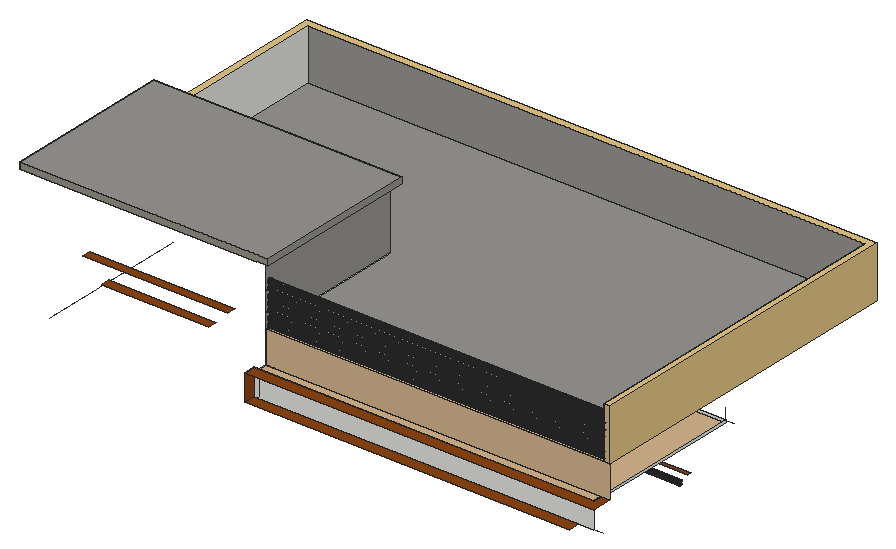
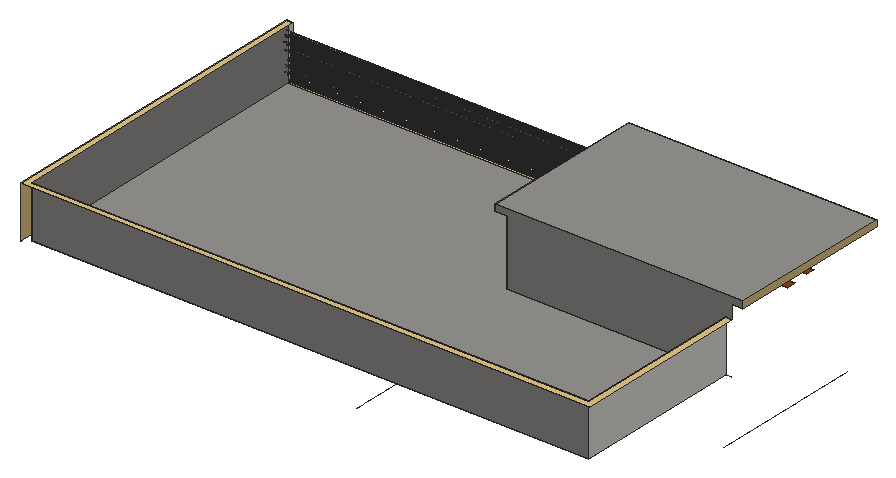
# SketchUp Ruby script. Lengths in inches.
U = 1.inch
M = Sketchup.active_model
def pt(a) = Geom::Point3d.new(a.map { |v| v * U })
def face(e, loops, mat)
  f = e.add_face(loops[0].map { |a| pt(a) })
  loops[1..].each { |l| e.add_face(l.map { |a| pt(a) }).erase! }
  f.material = f.back_material = mat if mat
  f
end
# faces: each face lists its corners as indices into pts; further lists are holes
def faces(e, pts, list, mat = nil) = list.each { |f| face(e, (f[0].is_a?(Array) ? f : [f]).map { |l| l.map { |i| pts[i] } }, mat) }
# xy, xz, yz: faces in a plane at the given z, y or x. An outline is a flat list of corners, or four numbers for a rectangle; further outlines are holes
def ring(l) = l.size == 4 ? [[l[0], l[1]], [l[2], l[1]], [l[2], l[3]], [l[0], l[3]]] : l.each_slice(2).to_a
def flat(e, list, mat, &to3) = list.each { |f| face(e, (f[0].is_a?(Array) ? f : [f]).map { |l| ring(l).map { |u, v| to3.(u, v) } }, mat) }
def xy(e, z, list, mat = nil) = flat(e, list, mat) { |x, y| [x, y, z] }
def xz(e, y, list, mat = nil) = flat(e, list, mat) { |x, z| [x, y, z] }
def yz(e, x, list, mat = nil) = flat(e, list, mat) { |y, z| [x, y, z] }
def lines(e, pts, list) = list.each { |a, b| e.add_line(pt(pts[a]), pt(pts[b])) }
# prism: a flat outline (further loops are holes) pulled along v
def prism(e, loops, v, mat = nil)
  f = face(e, loops, mat); d = Geom::Vector3d.new(v.map { |x| x * U })
  f.pushpull(f.normal.samedirection?(d) ? d.length : -d.length)
end
def box(e, o, s, mat = nil) = prism(e, [[o, [o[0] + s[0], o[1], o[2]], [o[0] + s[0], o[1] + s[1], o[2]], [o[0], o[1] + s[1], o[2]]]], [0, 0, s[2]], mat)
def at(x, y, z, deg = 0) = Geom::Transformation.translation(pt([x, y, z])) * Geom::Transformation.rotation(ORIGIN, Z_AXIS, deg.degrees)
def axes(o, x, y, z) = Geom::Transformation.new([*x, 0, *y, 0, *z, 0, *pt(o).to_a, 1])
def part(name) = M.definitions.add(name)
# library, detail: a bought-in or finely detailed component or shape, given as its bounding box
def library(name, o, s) = part(name).tap { |d| box(d.entities, o, s) }
def detail(e, o, s) = box(e.add_group.entities, o, s)
def put(e, d, t, mat = nil) = e.add_instance(d, t).tap { |i| i.material = mat if mat }
def group(e, t, mat = nil) = e.add_group.tap { |g| g.transformation = t; g.material = mat if mat }.entities
root = M.entities
M.materials.add("[0035_Tan]").color = [210, 180, 140]
M.materials.add("[0043_SaddleBrown]").color = [139, 69, 19]
M.materials.add("[Color M09]").color = [0, 0, 0]
M.materials.add("[Concrete Aggregate Smoke]").color = [154, 150, 148]
M.materials.add("[Formica Graystone]").color = [149, 146, 135]
M.materials.add("[Granite Light Gray]").color = [149, 148, 144]
M.materials.add("[Stone Brushed Khaki]").color = [226, 197, 133]
M.materials.add("[Terrazzo Tile Light]").color = [219, 217, 210]
M.materials.add("[Wood Lumber ButtJoined]").color = [164, 152, 112]
M.materials.add("[Wood Veneer 01]").color = [120, 70, 37]
xy(root,204,[[511.18,244.17,515.23,247.17]])
xy(root,204,[[473.23,244.17,511.18,247.17],[515.23,244.17,557.23,247.17]],"[Wood Veneer 01]")
xy(root,207.54,[[291.78,244.17,385.09,254.42]],"[Concrete Aggregate Smoke]")
xy(root,212.97,[[464.26,244.17,566.2,247.17]],"[Wood Veneer 01]")
xy(root,216.54,[[282.78,244.17,394.09,247.17]],"[Color M09]")
xy(root,248.36,[[244.11,62.42,587.04,74.42]],"[0043_SaddleBrown]")
xy(root,273.75,[[249.49,74.42,249.49,83.42,258.19,83.42,258.19,247.17,603,247.17,603,74.42]],"[0035_Tan]")
xy(root,276,[[249.49,83.42,257.61,247.17],[257.61,83.42,258.19,247.17]])
xy(root,276,[[249.49,74.42,603,83.42]],"[0035_Tan]")
xy(root,276,[[244.11,62.42,612,62.42,612,83.42,603,83.42,603,74.42,244.11,74.42]],"[0043_SaddleBrown]")
xy(root,297.68,[[83.36,74.42,196.9,83.42]],"[0043_SaddleBrown]")
xy(root,310.0625,[[612,83.42,612.4375,434.42]])
xy(root,310.0625,[[249.49,83.42,605.47,89.95]],"[0035_Tan]")
xy(root,310.0625,[[249.49,89.95,605.47,89.95,605.47,427.89,18.53,427.89,18.53,247.17,249.49,247.17]],"[Granite Light Gray]")
xy(root,317.69,[[63.35,74.42,216.91,83.42]],"[0043_SaddleBrown]")
xy(root,364.4375,[[605.47,83.42,612.4375,83.42,612.4375,434.42,12,434.42,12,247.17,18.53,247.17,18.53,427.89,605.47,427.89]],"[Stone Brushed Khaki]")
xy(root,378.52,[[12,71.42,249.49,83.42]],"[Formica Graystone]")
xy(root,378.73,[[0,71.42,12,247.17]],"[Stone Brushed Khaki]")
xy(root,379.14,[[249.49,71.42,261.49,247.17]],"[Granite Light Gray]")
xy(root,385.875,[[0,71.42,261.49,247.17]],"[Granite Light Gray]")
xz(root,71.42,[[12,378.52,249.49,378.52,249.49,379.14,261.49,379.14,261.49,385.875,0,385.875,0,378.73,12,378.73]],"[Formica Graystone]")
xz(root,74.42,[[244.11,248.36,249.49,273.75],[249.49,248.36,603,273.75],[244.11,273.75,249.49,276],[249.49,273.75,603,276]])
xz(root,83.42,[[249.49,273.75,257.61,276],[257.61,273.75,258.19,276]])
xz(root,83.42,[[249.49,276,612,310.0625],[605.47,310.0625,612.4375,364.4375]],"[0035_Tan]")
xz(root,247.17,[[258.19,273.75,603,276]])
xz(root,247.17,[[18.53,310.0625,18.53,364.4375,12,364.4375,12,378.73,0,378.73,0,385.875,261.49,385.875,261.49,379.14,249.49,379.14,249.49,310.0625]],"[Granite Light Gray]")
xz(root,427.89,[[18.53,310.0625,605.47,364.4375]],"[Granite Light Gray]")
yz(root,0,[[71.42,378.73,247.17,385.875]],"[Stone Brushed Khaki]")
yz(root,18.53,[[247.17,310.0625,427.89,364.4375]])
yz(root,244.11,[[62.42,248.36,74.42,276]],"[0043_SaddleBrown]")
yz(root,249.49,[[74.42,273.75,83.42,276],[[83.42,276,247.17,310.0625],[86.63,303.76,86.07,303.83,85.54,304.05,85.09,304.4,84.74,304.85,84.52,305.375,84.45,305.94,84.52,306.51,84.74,307.04,85.09,307.49,85.54,307.84,86.07,308.06,86.63,308.13,87.2,308.06,87.73,307.84,88.18,307.49,88.53,307.04,88.75,306.51,88.82,305.94,88.75,305.375,88.53,304.85,88.18,304.4,87.73,304.05,87.2,303.83],[86.63,296.82,86.07,296.89,85.54,297.11,85.09,297.46,84.74,297.91,84.52,298.4375,84.45,299.01,84.52,299.57,84.74,300.1,85.09,300.55,85.54,300.9,86.07,301.12,86.63,301.19,87.2,301.12,87.73,300.9,88.18,300.55,88.53,300.1,88.75,299.57,88.82,299.01,88.75,298.4375,88.53,297.91,88.18,297.46,87.73,297.11,87.2,296.89]],[86.63,296.82,87.2,296.89,87.73,297.11,88.18,297.46,88.53,297.91,88.75,298.4375,88.82,299.01,88.75,299.57,88.53,300.1,88.18,300.55,87.73,300.9,87.2,301.12,86.63,301.19,86.07,301.12,85.54,300.9,85.09,300.55,84.74,300.1,84.52,299.57,84.45,299.01,84.52,298.4375,84.74,297.91,85.09,297.46,85.54,297.11,86.07,296.89],[86.63,303.76,87.2,303.83,87.73,304.05,88.18,304.4,88.53,304.85,88.75,305.375,88.82,305.94,88.75,306.51,88.53,307.04,88.18,307.49,87.73,307.84,87.2,308.06,86.63,308.13,86.07,308.06,85.54,307.84,85.09,307.49,84.74,307.04,84.52,306.51,84.45,305.94,84.52,305.375,84.74,304.85,85.09,304.4,85.54,304.05,86.07,303.83]])
yz(root,249.49,[[[83.42,310.0625,247.17,310.0625,247.17,379.14,71.42,379.14,71.42,378.52,83.42,378.52],[86.63,345.38,86.07,345.45,85.54,345.67,85.09,346.02,84.74,346.47,84.52,347,84.45,347.57,84.52,348.13,84.74,348.66,85.09,349.11,85.54,349.46,86.07,349.68,86.63,349.76,87.2,349.68,87.73,349.46,88.18,349.11,88.53,348.66,88.75,348.13,88.82,347.57,88.75,347,88.53,346.47,88.18,346.02,87.73,345.67,87.2,345.45],[86.63,338.44,86.07,338.52,85.54,338.74,85.09,339.08,84.74,339.54,84.52,340.0625,84.45,340.63,84.52,341.2,84.74,341.72,85.09,342.18,85.54,342.52,86.07,342.74,86.63,342.82,87.2,342.74,87.73,342.52,88.18,342.18,88.53,341.72,88.75,341.2,88.82,340.63,88.75,340.0625,88.53,339.54,88.18,339.08,87.73,338.74,87.2,338.52],[86.63,331.51,86.07,331.58,85.54,331.8,85.09,332.15,84.74,332.6,84.52,333.125,84.45,333.69,84.52,334.26,84.74,334.79,85.09,335.24,85.54,335.59,86.07,335.81,86.63,335.88,87.2,335.81,87.73,335.59,88.18,335.24,88.53,334.79,88.75,334.26,88.82,333.69,88.75,333.125,88.53,332.6,88.18,332.15,87.73,331.8,87.2,331.58],[86.63,324.57,86.07,324.64,85.54,324.86,85.09,325.21,84.74,325.66,84.52,326.1875,84.45,326.76,84.52,327.32,84.74,327.85,85.09,328.3,85.54,328.65,86.07,328.87,86.63,328.94,87.2,328.87,87.73,328.65,88.18,328.3,88.53,327.85,88.75,327.32,88.82,326.76,88.75,326.1875,88.53,325.66,88.18,325.21,87.73,324.86,87.2,324.64],[86.63,317.63,86.07,317.7,85.54,317.92,85.09,318.27,84.74,318.72,84.52,319.25,84.45,319.82,84.52,320.38,84.74,320.91,85.09,321.36,85.54,321.71,86.07,321.93,86.63,322.01,87.2,321.93,87.73,321.71,88.18,321.36,88.53,320.91,88.75,320.38,88.82,319.82,88.75,319.25,88.53,318.72,88.18,318.27,87.73,317.92,87.2,317.7],[86.63,310.69,86.07,310.77,85.54,310.99,85.09,311.33,84.74,311.79,84.52,312.3125,84.45,312.88,84.52,313.45,84.74,313.97,85.09,314.43,85.54,314.77,86.07,314.99,86.63,315.07,87.2,314.99,87.73,314.77,88.18,314.43,88.53,313.97,88.75,313.45,88.82,312.88,88.75,312.3125,88.53,311.79,88.18,311.33,87.73,310.99,87.2,310.77],[86.63,352.32,86.07,352.39,85.54,352.61,85.09,352.96,84.74,353.41,84.52,353.9375,84.45,354.51,84.52,355.07,84.74,355.6,85.09,356.05,85.54,356.4,86.07,356.62,86.63,356.69,87.2,356.62,87.73,356.4,88.18,356.05,88.53,355.6,88.75,355.07,88.82,354.51,88.75,353.9375,88.53,353.41,88.18,352.96,87.73,352.61,87.2,352.39]]],"[Granite Light Gray]")
yz(root,258.19,[[83.42,273.75,247.17,276]])
yz(root,261.49,[[71.42,379.14,247.17,385.875]],"[Granite Light Gray]")
yz(root,386.65,[[249.32,200.85,249.99,200.94,250.6,201.2,251.14,201.6,251.54,202.13,251.8,202.75,251.89,203.42,251.8,204.08,251.54,204.7,251.14,205.23,250.6,205.63,249.99,205.89,249.32,205.98,248.66,205.89,248.04,205.63,247.51,205.23,247.1,204.7,246.85,204.08,246.76,203.42,246.85,202.75,247.1,202.13,247.51,201.6,248.04,201.2,248.66,200.94]])
yz(root,603,[[74.42,273.75,247.17,276]])
yz(root,605.47,[[83.42,310.0625,89.95,364.4375]])
yz(root,605.47,[[89.95,310.0625,427.89,364.4375]],"[Granite Light Gray]")
yz(root,610.02,[[86.63,310.69,87.2,310.77,87.73,310.99,88.18,311.33,88.53,311.79,88.75,312.3125,88.82,312.88,88.75,313.45,88.53,313.97,88.18,314.43,87.73,314.77,87.2,314.99,86.63,315.07,86.07,314.99,85.54,314.77,85.09,314.43,84.74,313.97,84.52,313.45,84.45,312.88,84.52,312.3125,84.74,311.79,85.09,311.33,85.54,310.99,86.07,310.77],[86.63,317.63,87.2,317.7,87.73,317.92,88.18,318.27,88.53,318.72,88.75,319.25,88.82,319.82,88.75,320.38,88.53,320.91,88.18,321.36,87.73,321.71,87.2,321.93,86.63,322.01,86.07,321.93,85.54,321.71,85.09,321.36,84.74,320.91,84.52,320.38,84.45,319.82,84.52,319.25,84.74,318.72,85.09,318.27,85.54,317.92,86.07,317.7],[86.63,324.57,87.2,324.64,87.73,324.86,88.18,325.21,88.53,325.66,88.75,326.1875,88.82,326.76,88.75,327.32,88.53,327.85,88.18,328.3,87.73,328.65,87.2,328.87,86.63,328.94,86.07,328.87,85.54,328.65,85.09,328.3,84.74,327.85,84.52,327.32,84.45,326.76,84.52,326.1875,84.74,325.66,85.09,325.21,85.54,324.86,86.07,324.64],[86.63,331.51,87.2,331.58,87.73,331.8,88.18,332.15,88.53,332.6,88.75,333.125,88.82,333.69,88.75,334.26,88.53,334.79,88.18,335.24,87.73,335.59,87.2,335.81,86.63,335.88,86.07,335.81,85.54,335.59,85.09,335.24,84.74,334.79,84.52,334.26,84.45,333.69,84.52,333.125,84.74,332.6,85.09,332.15,85.54,331.8,86.07,331.58]])
yz(root,612,[[86.63,338.44,87.2,338.52,87.73,338.74,88.18,339.08,88.53,339.54,88.75,340.0625,88.82,340.63,88.75,341.2,88.53,341.72,88.18,342.18,87.73,342.52,87.2,342.74,86.63,342.82,86.07,342.74,85.54,342.52,85.09,342.18,84.74,341.72,84.52,341.2,84.45,340.63,84.52,340.0625,84.74,339.54,85.09,339.08,85.54,338.74,86.07,338.52],[86.63,345.38,87.2,345.45,87.73,345.67,88.18,346.02,88.53,346.47,88.75,347,88.82,347.57,88.75,348.13,88.53,348.66,88.18,349.11,87.73,349.46,87.2,349.68,86.63,349.76,86.07,349.68,85.54,349.46,85.09,349.11,84.74,348.66,84.52,348.13,84.45,347.57,84.52,347,84.74,346.47,85.09,346.02,85.54,345.67,86.07,345.45],[86.63,352.32,87.2,352.39,87.73,352.61,88.18,352.96,88.53,353.41,88.75,353.9375,88.82,354.51,88.75,355.07,88.53,355.6,88.18,356.05,87.73,356.4,87.2,356.62,86.63,356.69,86.07,356.62,85.54,356.4,85.09,356.05,84.74,355.6,84.52,355.07,84.45,354.51,84.52,353.9375,84.74,353.41,85.09,352.96,85.54,352.61,86.07,352.39]])
yz(root,612.4375,[[83.42,310.0625,434.42,364.4375]],"[Stone Brushed Khaki]")
p = [[473.23,245.22,198.83],[473.23,245.45,198.73],[557.23,245.45,198.73],[557.23,245.22,198.83],[473.23,245.69,198.7],[557.23,245.69,198.7],
  [473.23,245.94,198.73],[557.23,245.94,198.73],[473.23,246.16,198.83],[557.23,246.16,198.83],[473.23,245.03,198.98],[557.23,245.03,198.98],
  [473.23,246.36,198.98],[557.23,246.36,198.98],[473.23,244.88,199.17],[557.23,244.88,199.17],[473.23,246.5,199.17],[557.23,246.5,199.17],
  [473.23,244.79,199.4],[557.23,244.79,199.4],[473.23,246.6,199.4],[557.23,246.6,199.4],[473.23,244.75,199.64],[557.23,244.75,199.64],
  [473.23,246.63,199.64],[557.23,246.63,199.64],[473.23,244.79,199.88],[557.23,244.79,199.88],[473.23,246.6,199.88],[557.23,246.6,199.88],
  [473.23,244.88,200.11],[557.23,244.88,200.11],[473.23,246.5,200.11],[557.23,246.5,200.11],[473.23,245.03,200.3],[557.23,245.03,200.3],
  [473.23,246.36,200.3],[557.23,246.36,200.3],[473.23,245.22,200.45],[557.23,245.22,200.45],[473.23,246.16,200.45],[557.23,246.16,200.45],
  [473.23,245.45,200.54],[557.23,245.45,200.54],[473.23,245.69,200.58],[557.23,245.69,200.58],[473.23,245.94,200.54],[557.23,245.94,200.54],
  [291.78,248.04,201.2],[291.78,248.66,200.94],[386.65,248.66,200.94],[386.65,248.04,201.2],[291.78,249.32,200.85],[386.65,249.32,200.85],
  [291.78,249.99,200.94],[386.65,249.99,200.94],[291.78,250.6,201.2],[386.65,250.6,201.2],[291.78,247.51,201.6],[386.65,247.51,201.6],
  [291.78,251.14,201.6],[386.65,251.14,201.6],[473.23,245.22,201.58],[473.23,245.45,201.48],[557.23,245.45,201.48],[557.23,245.22,201.58],
  [473.23,245.69,201.45],[557.23,245.69,201.45],[473.23,245.94,201.48],[557.23,245.94,201.48],[473.23,246.16,201.58],[557.23,246.16,201.58],
  [473.23,245.03,201.73],[557.23,245.03,201.73],[473.23,246.36,201.73],[557.23,246.36,201.73],[291.78,247.1,202.13],[386.65,247.1,202.13],
  [291.78,251.54,202.13],[386.65,251.54,202.13],[473.23,244.88,201.92],[557.23,244.88,201.92],[473.23,246.5,201.92],[557.23,246.5,201.92],
  [473.23,244.79,202.15],[557.23,244.79,202.15],[473.23,246.6,202.15],[557.23,246.6,202.15],[473.23,244.75,202.39],[557.23,244.75,202.39],
  [473.23,246.63,202.39],[557.23,246.63,202.39],[291.78,246.85,202.75],[386.65,246.85,202.75],[291.78,251.8,202.75],[386.65,251.8,202.75],
  [473.23,244.79,202.63],[557.23,244.79,202.63],[473.23,246.6,202.63],[557.23,246.6,202.63],[473.23,244.88,202.86],[557.23,244.88,202.86],
  [473.23,246.5,202.86],[557.23,246.5,202.86],[291.78,246.76,203.42],[386.65,246.76,203.42],[291.78,251.89,203.42],[386.65,251.89,203.42],
  [473.23,245.03,203.05],[557.23,245.03,203.05],[473.23,246.36,203.05],[557.23,246.36,203.05],[473.23,245.22,203.2],[557.23,245.22,203.2],
  [473.23,246.16,203.2],[557.23,246.16,203.2],[473.23,245.45,203.29],[557.23,245.45,203.29],[473.23,245.94,203.29],[557.23,245.94,203.29],
  [473.23,245.69,203.33],[557.23,245.69,203.33],[291.78,246.85,204.08],[386.65,246.85,204.08],[291.78,251.8,204.08],[386.65,251.8,204.08],
  [291.78,247.1,204.7],[386.65,247.1,204.7],[291.78,251.54,204.7],[386.65,251.54,204.7],[291.78,247.51,205.23],[386.65,247.51,205.23],
  [291.78,251.14,205.23],[386.65,251.14,205.23],[291.78,248.04,205.63],[386.65,248.04,205.63],[291.78,250.6,205.63],[386.65,250.6,205.63],
  [291.78,248.66,205.89],[386.65,248.66,205.89],[291.78,249.99,205.89],[386.65,249.99,205.89],[291.78,249.32,205.98],[386.65,249.32,205.98],
  [339.9,244.17,207.54],[338.43,244.17,207.54],[337.18,244.17,207.54],[337.18,241.18,207.41],[339.9,241.18,207.41],[249.49,86.07,310.77],
  [249.49,86.63,310.69],[610.02,86.63,310.69],[610.02,86.07,310.77],[249.49,87.2,310.77],[610.02,87.2,310.77],[249.49,85.54,310.99],
  [610.02,85.54,310.99],[249.49,87.73,310.99],[610.02,87.73,310.99],[249.49,85.09,311.33],[610.02,85.09,311.33],[249.49,88.18,311.33],
  [610.02,88.18,311.33],[249.49,84.74,311.79],[610.02,84.74,311.79],[249.49,88.53,311.79],[610.02,88.53,311.79],[249.49,84.52,312.3125],
  [610.02,84.52,312.3125],[249.49,88.75,312.3125],[610.02,88.75,312.3125],[249.49,84.45,312.88],[610.02,84.45,312.88],[249.49,88.82,312.88],
  [610.02,88.82,312.88],[249.49,84.52,313.45],[610.02,84.52,313.45],[249.49,88.75,313.45],[610.02,88.75,313.45],[249.49,84.74,313.97],
  [610.02,84.74,313.97],[249.49,88.53,313.97],[610.02,88.53,313.97],[249.49,85.09,314.43],[610.02,85.09,314.43],[249.49,88.18,314.43],
  [610.02,88.18,314.43],[249.49,85.54,314.77],[610.02,85.54,314.77],[249.49,87.73,314.77],[610.02,87.73,314.77],[249.49,86.07,314.99],
  [610.02,86.07,314.99],[249.49,87.2,314.99],[610.02,87.2,314.99],[249.49,86.63,315.07],[610.02,86.63,315.07],[249.49,86.07,317.7],
  [249.49,86.63,317.63],[610.02,86.63,317.63],[610.02,86.07,317.7],[249.49,87.2,317.7],[610.02,87.2,317.7],[249.49,85.54,317.92],
  [610.02,85.54,317.92],[249.49,87.73,317.92],[610.02,87.73,317.92],[249.49,85.09,318.27],[610.02,85.09,318.27],[249.49,88.18,318.27],
  [610.02,88.18,318.27],[249.49,84.74,318.72],[610.02,84.74,318.72],[249.49,88.53,318.72],[610.02,88.53,318.72],[249.49,84.52,319.25],
  [610.02,84.52,319.25],[249.49,88.75,319.25],[610.02,88.75,319.25],[249.49,84.45,319.82],[610.02,84.45,319.82],[249.49,88.82,319.82],
  [610.02,88.82,319.82],[249.49,84.52,320.38],[610.02,84.52,320.38],[249.49,88.75,320.38],[610.02,88.75,320.38],[249.49,84.74,320.91],
  [610.02,84.74,320.91],[249.49,88.53,320.91],[610.02,88.53,320.91],[249.49,85.09,321.36],[610.02,85.09,321.36],[249.49,88.18,321.36],
  [610.02,88.18,321.36],[249.49,85.54,321.71],[610.02,85.54,321.71],[249.49,87.73,321.71],[610.02,87.73,321.71],[249.49,86.07,321.93],
  [610.02,86.07,321.93],[249.49,87.2,321.93],[610.02,87.2,321.93],[249.49,86.63,322.01],[610.02,86.63,322.01],[249.49,85.54,324.86],
  [249.49,86.07,324.64],[610.02,86.07,324.64],[610.02,85.54,324.86],[249.49,86.63,324.57],[610.02,86.63,324.57],[249.49,87.2,324.64],
  [610.02,87.2,324.64],[249.49,87.73,324.86],[610.02,87.73,324.86],[249.49,85.09,325.21],[610.02,85.09,325.21],[249.49,88.18,325.21],
  [610.02,88.18,325.21],[249.49,84.74,325.66],[610.02,84.74,325.66],[249.49,88.53,325.66],[610.02,88.53,325.66],[249.49,84.52,326.1875],
  [610.02,84.52,326.1875],[249.49,88.75,326.1875],[610.02,88.75,326.1875],[249.49,84.45,326.76],[610.02,84.45,326.76],[249.49,88.82,326.76],
  [610.02,88.82,326.76],[249.49,84.52,327.32],[610.02,84.52,327.32],[249.49,88.75,327.32],[610.02,88.75,327.32],[249.49,84.74,327.85],
  [610.02,84.74,327.85],[249.49,88.53,327.85],[610.02,88.53,327.85],[249.49,85.09,328.3],[610.02,85.09,328.3],[249.49,88.18,328.3],
  [610.02,88.18,328.3],[249.49,85.54,328.65],[610.02,85.54,328.65],[249.49,87.73,328.65],[610.02,87.73,328.65],[249.49,86.07,328.87],
  [610.02,86.07,328.87],[249.49,87.2,328.87],[610.02,87.2,328.87],[249.49,86.63,328.94],[610.02,86.63,328.94],[249.49,86.07,331.58],
  [249.49,86.63,331.51],[610.02,86.63,331.51],[610.02,86.07,331.58],[249.49,87.2,331.58],[610.02,87.2,331.58],[249.49,85.54,331.8],
  [610.02,85.54,331.8],[249.49,87.73,331.8],[610.02,87.73,331.8],[249.49,85.09,332.15],[610.02,85.09,332.15],[249.49,88.18,332.15],
  [610.02,88.18,332.15],[249.49,84.74,332.6],[610.02,84.74,332.6],[249.49,88.53,332.6],[610.02,88.53,332.6],[249.49,84.52,333.125],
  [610.02,84.52,333.125],[249.49,88.75,333.125],[610.02,88.75,333.125],[249.49,84.45,333.69],[610.02,84.45,333.69],[249.49,88.82,333.69],
  [610.02,88.82,333.69],[249.49,84.52,334.26],[610.02,84.52,334.26],[249.49,88.75,334.26],[610.02,88.75,334.26],[249.49,84.74,334.79],
  [610.02,84.74,334.79],[249.49,88.53,334.79],[610.02,88.53,334.79],[249.49,85.09,335.24],[610.02,85.09,335.24],[249.49,88.18,335.24],
  [610.02,88.18,335.24],[249.49,85.54,335.59],[610.02,85.54,335.59],[249.49,87.73,335.59],[610.02,87.73,335.59],[249.49,86.07,335.81],
  [610.02,86.07,335.81],[249.49,87.2,335.81],[610.02,87.2,335.81],[249.49,86.63,335.88],[610.02,86.63,335.88],[249.49,86.07,338.52],
  [249.49,86.63,338.44],[612,86.63,338.44],[612,86.07,338.52],[249.49,87.2,338.52],[612,87.2,338.52],[249.49,85.54,338.74],
  [612,85.54,338.74],[249.49,87.73,338.74],[612,87.73,338.74],[249.49,85.09,339.08],[612,85.09,339.08],[249.49,88.18,339.08],
  [612,88.18,339.08],[249.49,84.74,339.54],[612,84.74,339.54],[249.49,88.53,339.54],[612,88.53,339.54],[249.49,84.52,340.0625],
  [612,84.52,340.0625],[249.49,88.75,340.0625],[612,88.75,340.0625],[249.49,84.45,340.63],[612,84.45,340.63],[249.49,88.82,340.63],
  [612,88.82,340.63],[249.49,84.52,341.2],[612,84.52,341.2],[249.49,88.75,341.2],[612,88.75,341.2],[249.49,84.74,341.72],
  [612,84.74,341.72],[249.49,88.53,341.72],[612,88.53,341.72],[249.49,85.09,342.18],[612,85.09,342.18],[249.49,88.18,342.18],
  [612,88.18,342.18],[249.49,85.54,342.52],[612,85.54,342.52],[249.49,87.73,342.52],[612,87.73,342.52],[249.49,86.07,342.74],
  [612,86.07,342.74],[249.49,87.2,342.74],[612,87.2,342.74],[249.49,86.63,342.82],[612,86.63,342.82],[249.49,86.07,345.45],
  [249.49,86.63,345.38],[612,86.63,345.38],[612,86.07,345.45],[249.49,87.2,345.45],[612,87.2,345.45],[249.49,85.54,345.67],
  [612,85.54,345.67],[249.49,87.73,345.67],[612,87.73,345.67],[249.49,85.09,346.02],[612,85.09,346.02],[249.49,88.18,346.02],
  [612,88.18,346.02],[249.49,84.74,346.47],[612,84.74,346.47],[249.49,88.53,346.47],[612,88.53,346.47],[249.49,84.52,347],
  [612,84.52,347],[249.49,88.75,347],[612,88.75,347],[249.49,84.45,347.57],[612,84.45,347.57],[249.49,88.82,347.57],
  [612,88.82,347.57],[249.49,84.52,348.13],[612,84.52,348.13],[249.49,88.75,348.13],[612,88.75,348.13],[249.49,84.74,348.66],
  [612,84.74,348.66],[249.49,88.53,348.66],[612,88.53,348.66],[249.49,85.09,349.11],[612,85.09,349.11],[249.49,88.18,349.11],
  [612,88.18,349.11],[249.49,85.54,349.46],[612,85.54,349.46],[249.49,87.73,349.46],[612,87.73,349.46],[249.49,86.07,349.68],
  [612,86.07,349.68],[249.49,87.2,349.68],[612,87.2,349.68],[249.49,86.63,349.76],[612,86.63,349.76],[249.49,86.07,352.39],
  [249.49,86.63,352.32],[612,86.63,352.32],[612,86.07,352.39],[249.49,87.2,352.39],[612,87.2,352.39],[249.49,85.54,352.61],
  [612,85.54,352.61],[249.49,87.73,352.61],[612,87.73,352.61],[249.49,85.09,352.96],[612,85.09,352.96],[249.49,88.18,352.96],
  [612,88.18,352.96],[249.49,84.74,353.41],[612,84.74,353.41],[249.49,88.53,353.41],[612,88.53,353.41],[249.49,84.52,353.9375],
  [612,84.52,353.9375],[249.49,88.75,353.9375],[612,88.75,353.9375],[249.49,84.45,354.51],[612,84.45,354.51],[249.49,88.82,354.51],
  [612,88.82,354.51],[249.49,84.52,355.07],[612,84.52,355.07],[249.49,88.75,355.07],[612,88.75,355.07],[249.49,84.74,355.6],
  [612,84.74,355.6],[249.49,88.53,355.6],[612,88.53,355.6],[249.49,85.09,356.05],[612,85.09,356.05],[249.49,88.18,356.05],
  [612,88.18,356.05],[249.49,85.54,356.4],[612,85.54,356.4],[249.49,87.73,356.4],[612,87.73,356.4],[249.49,86.07,356.62],
  [612,86.07,356.62],[249.49,87.2,356.62],[612,87.2,356.62],[249.49,86.63,356.69],[612,86.63,356.69],[603,74.42,248.36],
  [612,74.42,248.36],[603,247.17,288],[603,247.17,276],[612,247.17,276],[250.05,83.42,288],[250.05,83.42,276],
  [21,247.17,240],[21,83.42,240],[258.19,247.17,276],[258.19,434.42,276],[18.53,247.17,310.0625],[12,247.17,310.0625]]
faces(root,p,[[0,1,2,3],[1,4,5,2],[4,6,7,5],[6,8,9,7],[10,0,3,11],[8,12,13,9],[14,10,11,15],[12,16,17,13],
  [18,14,15,19],[16,20,21,17],[22,18,19,23],[20,24,25,21],[26,22,23,27],[24,28,29,25],[30,26,27,31],[28,32,33,29],
  [34,30,31,35],[32,36,37,33],[38,34,35,39],[36,40,41,37],[42,38,39,43],[44,42,43,45],[46,44,45,47],[40,46,47,41],
  [62,63,64,65],[63,66,67,64],[66,68,69,67],[68,70,71,69],[72,62,65,73],[70,74,75,71],[80,72,73,81],[74,82,83,75],
  [84,80,81,85],[82,86,87,83],[88,84,85,89],[86,90,91,87],[96,88,89,97],[90,98,99,91],[100,96,97,101],[98,102,103,99],
  [108,100,101,109],[102,110,111,103],[112,108,109,113],[110,114,115,111],[116,112,113,117],[114,118,119,115],[120,116,117,121],[118,120,121,119]],"[Terrazzo Tile Light]")
faces(root,p,[[48,49,50,51],[49,52,53,50],[52,54,55,53],[54,56,57,55],[58,48,51,59],[56,60,61,57],[76,58,59,77],[60,78,79,61],
  [92,76,77,93],[78,94,95,79],[104,92,93,105],[94,106,107,95],[122,104,105,123],[106,124,125,107],[126,122,123,127],[124,128,129,125],
  [130,126,127,131],[128,132,133,129],[134,130,131,135],[132,136,137,133],[138,134,135,139],[136,140,141,137],[142,138,139,143],[140,142,143,141]],"[Wood Lumber ButtJoined]")
faces(root,p,[[144,145,146,147,148]])
faces(root,p,[[149,150,151,152],[150,153,154,151],[155,149,152,156],[153,157,158,154],[159,155,156,160],[157,161,162,158],[163,159,160,164],[161,165,166,162],
  [167,163,164,168],[165,169,170,166],[171,167,168,172],[169,173,174,170],[175,171,172,176],[173,177,178,174],[179,175,176,180],[177,181,182,178],
  [183,179,180,184],[181,185,186,182],[187,183,184,188],[185,189,190,186],[191,187,188,192],[189,193,194,190],[195,191,192,196],[193,195,196,194],
  [197,198,199,200],[198,201,202,199],[203,197,200,204],[201,205,206,202],[207,203,204,208],[205,209,210,206],[211,207,208,212],[209,213,214,210],
  [215,211,212,216],[213,217,218,214],[219,215,216,220],[217,221,222,218],[223,219,220,224],[221,225,226,222],[227,223,224,228],[225,229,230,226],
  [231,227,228,232],[229,233,234,230],[235,231,232,236],[233,237,238,234],[239,235,236,240],[237,241,242,238],[243,239,240,244],[241,243,244,242],
  [245,246,247,248],[246,249,250,247],[249,251,252,250],[251,253,254,252],[255,245,248,256],[253,257,258,254],[259,255,256,260],[257,261,262,258],
  [263,259,260,264],[261,265,266,262],[267,263,264,268],[265,269,270,266],[271,267,268,272],[269,273,274,270],[275,271,272,276],[273,277,278,274],
  [279,275,276,280],[277,281,282,278],[283,279,280,284],[281,285,286,282],[287,283,284,288],[285,289,290,286],[291,287,288,292],[289,291,292,290],
  [293,294,295,296],[294,297,298,295],[299,293,296,300],[297,301,302,298],[303,299,300,304],[301,305,306,302],[307,303,304,308],[305,309,310,306],
  [311,307,308,312],[309,313,314,310],[315,311,312,316],[313,317,318,314],[319,315,316,320],[317,321,322,318],[323,319,320,324],[321,325,326,322],
  [327,323,324,328],[325,329,330,326],[331,327,328,332],[329,333,334,330],[335,331,332,336],[333,337,338,334],[339,335,336,340],[337,339,340,338],
  [341,342,343,344],[342,345,346,343],[347,341,344,348],[345,349,350,346],[351,347,348,352],[349,353,354,350],[355,351,352,356],[353,357,358,354],
  [359,355,356,360],[357,361,362,358],[363,359,360,364],[361,365,366,362],[367,363,364,368],[365,369,370,366],[371,367,368,372],[369,373,374,370],
  [375,371,372,376],[373,377,378,374],[379,375,376,380],[377,381,382,378],[383,379,380,384],[381,385,386,382],[387,383,384,388],[385,387,388,386],
  [389,390,391,392],[390,393,394,391],[395,389,392,396],[393,397,398,394],[399,395,396,400],[397,401,402,398],[403,399,400,404],[401,405,406,402],
  [407,403,404,408],[405,409,410,406],[411,407,408,412],[409,413,414,410],[415,411,412,416],[413,417,418,414],[419,415,416,420],[417,421,422,418],
  [423,419,420,424],[421,425,426,422],[427,423,424,428],[425,429,430,426],[431,427,428,432],[429,433,434,430],[435,431,432,436],[433,435,436,434],
  [437,438,439,440],[438,441,442,439],[443,437,440,444],[441,445,446,442],[447,443,444,448],[445,449,450,446],[451,447,448,452],[449,453,454,450],
  [455,451,452,456],[453,457,458,454],[459,455,456,460],[457,461,462,458],[463,459,460,464],[461,465,466,462],[467,463,464,468],[465,469,470,466],
  [471,467,468,472],[469,473,474,470],[475,471,472,476],[473,477,478,474],[479,475,476,480],[477,481,482,478],[483,479,480,484],[481,483,484,482]],"[Concrete Aggregate Smoke]")
lines(root,p,[[485,486],[487,488],[488,489],[490,491],[492,493],[494,495],[496,497]])
